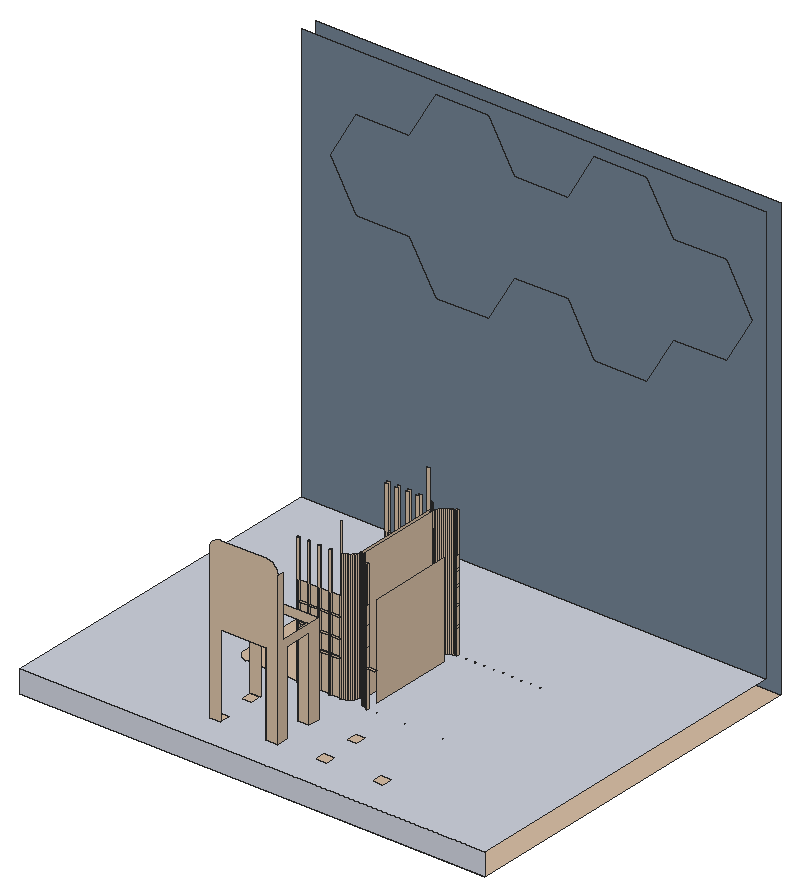
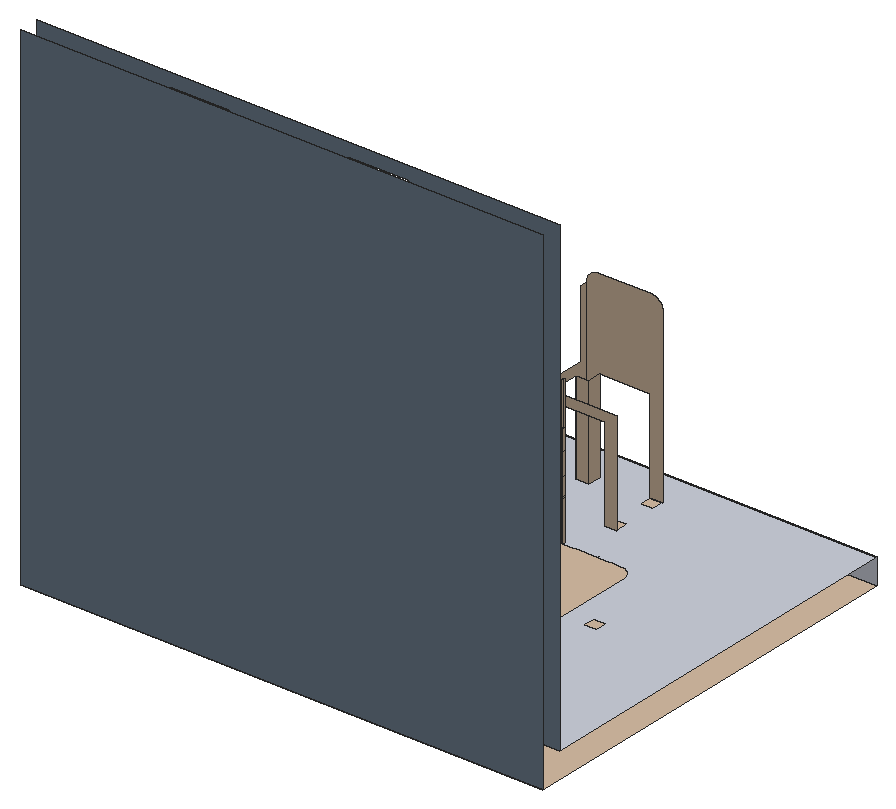
# SketchUp Ruby script. Lengths in inches.
U = 1.inch
M = Sketchup.active_model
def pt(a) = Geom::Point3d.new(a.map { |v| v * U })
def face(e, loops, mat)
  f = e.add_face(loops[0].map { |a| pt(a) })
  loops[1..].each { |l| e.add_face(l.map { |a| pt(a) }).erase! }
  f.material = f.back_material = mat if mat
  f
end
# faces: each face lists its corners as indices into pts; further lists are holes
def faces(e, pts, list, mat = nil) = list.each { |f| face(e, (f[0].is_a?(Array) ? f : [f]).map { |l| l.map { |i| pts[i] } }, mat) }
# xy, xz, yz: faces in a plane at the given z, y or x. An outline is a flat list of corners, or four numbers for a rectangle; further outlines are holes
def ring(l) = l.size == 4 ? [[l[0], l[1]], [l[2], l[1]], [l[2], l[3]], [l[0], l[3]]] : l.each_slice(2).to_a
def flat(e, list, mat, &to3) = list.each { |f| face(e, (f[0].is_a?(Array) ? f : [f]).map { |l| ring(l).map { |u, v| to3.(u, v) } }, mat) }
def xy(e, z, list, mat = nil) = flat(e, list, mat) { |x, y| [x, y, z] }
def xz(e, y, list, mat = nil) = flat(e, list, mat) { |x, z| [x, y, z] }
def yz(e, x, list, mat = nil) = flat(e, list, mat) { |y, z| [x, y, z] }
def lines(e, pts, list) = list.each { |a, b| e.add_line(pt(pts[a]), pt(pts[b])) }
# prism: a flat outline (further loops are holes) pulled along v
def prism(e, loops, v, mat = nil)
  f = face(e, loops, mat); d = Geom::Vector3d.new(v.map { |x| x * U })
  f.pushpull(f.normal.samedirection?(d) ? d.length : -d.length)
end
def box(e, o, s, mat = nil) = prism(e, [[o, [o[0] + s[0], o[1], o[2]], [o[0] + s[0], o[1] + s[1], o[2]], [o[0], o[1] + s[1], o[2]]]], [0, 0, s[2]], mat)
def at(x, y, z, deg = 0) = Geom::Transformation.translation(pt([x, y, z])) * Geom::Transformation.rotation(ORIGIN, Z_AXIS, deg.degrees)
def axes(o, x, y, z) = Geom::Transformation.new([*x, 0, *y, 0, *z, 0, *pt(o).to_a, 1])
def part(name) = M.definitions.add(name)
# library, detail: a bought-in or finely detailed component or shape, given as its bounding box
def library(name, o, s) = part(name).tap { |d| box(d.entities, o, s) }
def detail(e, o, s) = box(e.add_group.entities, o, s)
def put(e, d, t, mat = nil) = e.add_instance(d, t).tap { |i| i.material = mat if mat }
def group(e, t, mat = nil) = e.add_group.tap { |g| g.transformation = t; g.material = mat if mat }.entities
root = M.entities
M.materials.add("[0111_SlateGray]").color = [112, 128, 144]
M.materials.add("[Formica Laminate Light]").color = [213, 189, 164]
M.materials.add("[Marble Carrara Floor Tile]").color = [204, 208, 219]
xy(root,-6.9375,[[214.53,88,358.53,202.625]],"[Formica Laminate Light]")
xy(root,0,[[292.27,124.79,292.63,125.33],[270.89,124.84,271.32,125.33],[274.19,124.84,274.625,125.33],[277.49,124.84,277.93,125.33],[280.8,124.84,281.23,125.33],
  [284.1,124.84,284.53,125.33],[270.69,159.08,271.5,160.01],[273.95,159.08,274.76,160.01],[277.21,159.08,278.02,160.01],[280.47,159.08,281.29,160.01],
  [283.74,159.08,284.55,160.01],[292.34,159.08,293.16,159.77]],"[Formica Laminate Light]")
xy(root,0,[[[214.53,88,358.53,197],[254.37,124.84,254.37,125.33,254.38,125.33,253.95,125.44,253.54,125.6,253.14,125.79,252.77,126.03,252.42,126.3,252.09,126.61,251.81,126.95,251.55,127.3125,251.34,127.7,251.16,128.11,251.03,128.53,250.94,128.96,250.94,156.11,251.04,156.5625,251.21,157.03,251.45,157.47,251.74,157.87,252.09,158.22,252.49,158.52,252.93,158.76,253.4,158.94,253.88,159.05,254.38,159.08,254.38,160.01,255.19,160.01,255.19,159.08,257.64,159.08,257.64,160.01,258.46,160.01,258.46,159.08,260.91,159.08,260.91,160.01,261.72,160.01,261.72,159.08,264.17,159.08,264.17,160.01,264.98,160.01,264.98,159.08,267.43,159.08,267.43,160.01,268.24,160.01,268.24,159.08,270.69,159.08,270.69,160.01,271.5,160.01,271.5,159.08,273.95,159.08,273.95,160.01,274.76,160.01,274.76,159.08,277.21,159.08,277.21,160.01,278.02,160.01,278.02,159.08,280.47,159.08,280.47,160.01,281.29,160.01,281.29,159.08,283.74,159.08,283.74,160.01,284.55,160.01,284.55,159.08,284.99,158.95,285.41,158.77,285.8125,158.55,286.1875,158.28,286.53,157.98,286.83,157.63,287.1,157.26,287.32,156.86,287.49,156.43,287.62,155.99,287.7,155.54,287.72,155.08,287.72,128.96,287.69,128.53,287.62,128.09,287.49,127.67,287.31,127.27,287.08,126.89,286.8125,126.55,286.5,126.23,286.16,125.96,285.78,125.73,285.38,125.55,284.96,125.41,284.53,125.33,284.53,124.84,284.1,124.84,284.1,125.33,281.23,125.33,281.23,124.84,280.8,124.84,280.8,125.33,277.93,125.33,277.93,124.84,277.49,124.84,277.49,125.33,274.625,125.33,274.625,124.84,274.19,124.84,274.19,125.33,271.32,125.33,271.32,124.84,270.89,124.84,270.89,125.33,268.02,125.33,268.02,124.84,267.58,124.84,267.58,125.33,264.71,125.33,264.71,124.84,264.28,124.84,264.28,125.33,261.41,125.33,261.41,124.84,260.98,124.84,260.98,125.33,258.11,125.33,258.11,124.84,257.68,124.84,257.68,125.33,254.81,125.33,254.81,124.84],[297.89,97.95,301.53,101.59],[315.45,97.95,319.1,101.59],[282.83,110.07,286.47,113.72],[282.83,97.95,286.47,101.59],[265.27,97.95,268.91,101.59],[297.89,110.07,301.35,113.72],[265.27,110.07,268.72,113.72],[241.57,147.05,245.21,150.5],[295.2,159.08,296.03,159.77],[318.11,159.08,318.9375,159.77],[292.34,159.08,293.16,159.77],[312.38,159.08,313.21,159.77],[300.93,159.08,301.75,159.77],[309.52,159.08,310.35,159.77],[315.25,159.08,316.07,159.77],[306.66,159.08,307.48,159.77],[298.0625,159.08,298.89,159.77],[303.79,159.08,304.62,159.77],[312.73,124.79,313.09,125.33],[309.81,124.79,310.17,125.33],[315.65,124.79,316.01,125.33],[298.11,124.79,298.47,125.33],[318.58,124.79,318.9375,125.33],[306.88,124.79,307.24,125.33],[295.1875,124.79,295.55,125.33],[301.04,124.79,301.4,125.33],[292.27,124.79,292.63,125.33],[303.96,124.79,304.32,125.33]]],"[Marble Carrara Floor Tile]")
xy(root,7.64,[[271.5,159.08,273.95,160.01],[274.76,159.08,277.21,160.01],[278.02,159.08,280.47,160.01],[281.29,159.08,283.74,160.01]],"[Formica Laminate Light]")
xy(root,8.44,[[271.5,159.08,273.95,160.01],[274.76,159.08,277.21,160.01],[278.02,159.08,280.47,160.01],[281.29,159.08,283.74,160.01]],"[Formica Laminate Light]")
xy(root,11.02,[[271.32,124.84,274.19,125.33],[274.625,124.84,277.49,125.33],[277.93,124.84,280.8,125.33],[281.23,124.84,284.1,125.33]],"[Formica Laminate Light]")
xy(root,11.55,[[292.63,124.79,295.1875,125.33],[271.32,124.84,274.19,125.33],[274.625,124.84,277.49,125.33],[277.93,124.84,280.8,125.33],[281.23,124.84,284.1,125.33]],"[Formica Laminate Light]")
xy(root,15.1,[[271.5,159.08,273.95,160.01],[274.76,159.08,277.21,160.01],[278.02,159.08,280.47,160.01],[281.29,159.08,283.74,160.01]],"[Formica Laminate Light]")
xy(root,15.9,[[271.5,159.08,273.95,160.01],[274.76,159.08,277.21,160.01],[278.02,159.08,280.47,160.01],[281.29,159.08,283.74,160.01]],"[Formica Laminate Light]")
xy(root,16.52,[[271.32,124.84,274.19,125.33],[274.625,124.84,277.49,125.33],[277.93,124.84,280.8,125.33],[281.23,124.84,284.1,125.33]],"[Formica Laminate Light]")
xy(root,20.88,[[271.5,159.08,273.95,160.01],[274.76,159.08,277.21,160.01],[278.02,159.08,280.47,160.01],[281.29,159.08,283.74,160.01]],"[Formica Laminate Light]")
xy(root,21.68,[[271.5,159.08,273.95,160.01],[274.76,159.08,277.21,160.01],[278.02,159.08,280.47,160.01],[281.29,159.08,283.74,160.01]],"[Formica Laminate Light]")
xy(root,22.54,[[271.32,124.84,274.19,125.33],[274.625,124.84,277.49,125.33],[277.93,124.84,280.8,125.33],[281.23,124.84,284.1,125.33]],"[Formica Laminate Light]")
xz(root,88,[[214.53,-6.9375,358.53,0]],"[Marble Carrara Floor Tile]")
xz(root,97.95,[[265.27,0,268.91,0,268.91,25.5625,282.83,25.5625,282.83,0,286.47,0,286.47,46.86,286.41,47.34,286.29,47.8,286.11,48.25,285.88,48.67,285.6,49.05,285.27,49.4,284.9,49.71,284.5,49.97,284.0625,50.17,283.61,50.32,283.14,50.41,282.66,50.4375,268.95,50.4375,268.47,50.41,268,50.3125,267.54,50.16,267.11,49.94,266.71,49.68,266.35,49.36,266.03,48.99,265.76,48.59,265.55,48.16,265.39,47.7,265.3,47.23,265.27,46.75]],"[Formica Laminate Light]")
xz(root,101.59,[[282.83,0,286.47,25.5625]],"[Formica Laminate Light]")
xz(root,110.07,[[282.83,0,286.47,25.5625]],"[Formica Laminate Light]")
xz(root,113.72,[[265.27,0,265.27,28.25,286.47,28.25,286.47,0,282.83,0,282.83,25.5625,268.72,25.5625,268.72,0]],"[Formica Laminate Light]")
xz(root,124.79,[[292.27,0,292.63,40.33]],"[Formica Laminate Light]")
xz(root,124.84,[[270.89,0,271.32,40.33],[274.19,0,274.625,40.33],[277.49,0,277.93,40.33],[280.8,0,281.23,40.33],[271.32,11.02,274.19,11.55],
  [274.625,11.02,277.49,11.55],[277.93,11.02,280.8,11.55],[281.23,11.02,284.1,11.55],[271.32,16.52,274.19,17.06],[274.625,16.52,277.49,17.06],
  [277.93,16.52,280.8,17.06],[281.23,16.52,284.1,17.06],[271.32,22.54,274.19,23.07],[274.625,22.54,277.49,23.07],[277.93,22.54,280.8,23.07],
  [281.23,22.54,284.1,23.07]],"[Formica Laminate Light]")
xz(root,125.33,[[270.89,0,271.32,11.02],[271.32,0,274.19,11.02],[274.19,0,274.625,11.02],[274.625,0,277.49,11.02],[277.49,0,277.93,11.02],
  [277.93,0,280.8,11.02],[280.8,0,281.23,11.02],[281.23,0,284.1,11.02],[284.1,0,284.1,11.02,281.23,11.02,281.23,11.55,284.1,11.55,284.1,49.31,284.53,49.31,284.53,0],[292.27,0,292.32,11.02],
  [292.32,0,292.63,11.02],[270.89,11.02,271.32,40.33],[274.19,11.02,274.625,40.33],[277.49,11.02,277.93,40.33],[280.8,11.02,281.23,40.33],
  [292.27,11.02,292.32,11.55],[292.32,11.02,292.63,11.55],[271.32,11.55,274.19,16.52],[274.625,11.55,277.49,16.52],[277.93,11.55,280.8,16.52],
  [281.23,11.55,284.1,16.52],[292.27,11.55,292.32,40.33],[292.32,11.55,292.63,40.33],[271.32,16.52,274.19,22.54],[274.625,16.52,277.49,22.54],
  [277.93,16.52,280.8,22.54],[281.23,16.52,284.1,22.54],[271.32,22.54,274.19,28.4],[274.625,22.54,277.49,28.4],[277.93,22.54,280.8,28.4],
  [281.23,22.54,284.1,28.4]],"[Formica Laminate Light]")
xz(root,159.08,[[270.69,0,271.5,40.33],[271.5,0,273.95,7.64],[273.95,0,274.76,40.33],[274.76,0,277.21,7.64],[277.21,0,278.02,40.33],
  [278.02,0,280.47,7.64],[280.47,0,281.29,40.33],[281.29,0,283.74,7.64],[283.74,0,284.55,0,284.55,49.31,283.74,49.31,283.74,8.44,281.29,8.44,281.29,7.64,283.74,7.64],[292.34,0,292.97,40.33],
  [292.97,0,293.16,40.33],[271.5,8.44,273.95,15.1],[274.76,8.44,277.21,15.1],[278.02,8.44,280.47,15.1],[281.29,8.44,283.74,15.1],
  [271.5,15.1,273.95,15.9],[274.76,15.1,277.21,15.9],[278.02,15.1,280.47,15.9],[281.29,15.1,283.74,15.9],[271.5,15.9,273.95,20.88],
  [274.76,15.9,277.21,20.88],[278.02,15.9,280.47,20.88],[281.29,15.9,283.74,20.88],[271.5,20.88,273.95,21.68],[274.76,20.88,277.21,21.68],
  [278.02,20.88,280.47,21.68],[281.29,20.88,283.74,21.68],[271.5,21.68,273.95,26.83],[274.76,21.68,277.21,26.83],[278.02,21.68,280.47,26.83],
  [281.29,21.68,283.74,26.83]],"[Formica Laminate Light]")
xz(root,159.77,[[292.34,0,293.16,40.33]],"[Formica Laminate Light]")
xz(root,160.01,[[270.69,0,271.5,40.33],[273.95,0,274.76,40.33],[277.21,0,278.02,40.33],[280.47,0,281.29,40.33],[271.5,7.64,273.95,8.44],
  [274.76,7.64,277.21,8.44],[278.02,7.64,280.47,8.44],[281.29,7.64,283.74,8.44],[271.5,15.1,273.95,15.9],[274.76,15.1,277.21,15.9],
  [278.02,15.1,280.47,15.9],[281.29,15.1,283.74,15.9],[271.5,20.88,273.95,21.68],[274.76,20.88,277.21,21.68],[278.02,20.88,280.47,21.68],
  [281.29,20.88,283.74,21.68]],"[Formica Laminate Light]")
xz(root,197,[[[214.53,0,358.53,129.75],[256.11,69.64,247.92,83.83,231.54,83.83,223.35,98.02,231.54,112.21,247.92,112.21,256.11,126.39,272.5,126.39,280.6875,112.21,297.07,112.21,305.26,126.39,321.64,126.39,329.84,112.21,346.22,112.21,354.41,98.02,346.22,83.83,329.84,83.83,321.64,69.64,305.26,69.64,297.07,83.83,280.6875,83.83,272.5,69.64]]],"[0111_SlateGray]")
xz(root,202.625,[[214.53,-6.9375,358.53,129.75]],"[0111_SlateGray]")
yz(root,270.69,[[159.08,0,160.01,7.64],[159.08,20.88,160.01,21.68],[159.08,21.68,160.01,26.83]],"[Formica Laminate Light]")
yz(root,270.89,[[124.84,0,125.33,11.02],[124.84,11.02,125.33,11.55],[124.84,11.55,125.33,16.52],[124.84,16.52,125.33,22.54],[124.84,22.54,125.33,28.4]],"[Formica Laminate Light]")
yz(root,271.32,[[124.84,0,125.33,11.02],[124.84,11.02,125.33,11.55],[124.84,11.55,125.33,16.52],[124.84,16.52,125.33,22.54],[124.84,22.54,125.33,28.4]],"[Formica Laminate Light]")
yz(root,271.5,[[159.08,0,160.01,7.64],[159.08,7.64,160.01,8.44],[159.08,8.44,160.01,15.1],[159.08,15.1,160.01,15.9],[159.08,15.9,160.01,20.88],
  [159.08,20.88,160.01,21.68],[159.08,21.68,160.01,26.83]],"[Formica Laminate Light]")
yz(root,273.95,[[159.08,0,160.01,7.64],[159.08,7.64,160.01,8.44],[159.08,8.44,160.01,15.1],[159.08,15.1,160.01,15.9],[159.08,15.9,160.01,20.88],
  [159.08,20.88,160.01,21.68],[159.08,21.68,160.01,26.83]],"[Formica Laminate Light]")
yz(root,274.19,[[124.84,0,125.33,11.02],[124.84,11.02,125.33,11.55],[124.84,11.55,125.33,16.52],[124.84,16.52,125.33,22.54],[124.84,22.54,125.33,28.4]],"[Formica Laminate Light]")
yz(root,274.625,[[124.84,0,125.33,11.02],[124.84,11.02,125.33,11.55],[124.84,11.55,125.33,16.52],[124.84,16.52,125.33,22.54],[124.84,22.54,125.33,28.4]],"[Formica Laminate Light]")
yz(root,274.76,[[159.08,0,160.01,7.64],[159.08,7.64,160.01,8.44],[159.08,8.44,160.01,15.1],[159.08,15.1,160.01,15.9],[159.08,15.9,160.01,20.88],
  [159.08,20.88,160.01,21.68],[159.08,21.68,160.01,26.83]],"[Formica Laminate Light]")
yz(root,277.21,[[159.08,0,160.01,7.64],[159.08,7.64,160.01,8.44],[159.08,8.44,160.01,15.1],[159.08,15.1,160.01,15.9],[159.08,15.9,160.01,20.88],
  [159.08,20.88,160.01,21.68],[159.08,21.68,160.01,26.83]],"[Formica Laminate Light]")
yz(root,277.49,[[124.84,0,125.33,11.02],[124.84,11.02,125.33,11.55],[124.84,11.55,125.33,16.52],[124.84,16.52,125.33,22.54],[124.84,22.54,125.33,28.4]],"[Formica Laminate Light]")
yz(root,277.93,[[124.84,0,125.33,11.02],[124.84,11.02,125.33,11.55],[124.84,11.55,125.33,16.52],[124.84,16.52,125.33,22.54],[124.84,22.54,125.33,28.4]],"[Formica Laminate Light]")
yz(root,278.02,[[159.08,0,160.01,7.64],[159.08,7.64,160.01,8.44],[159.08,8.44,160.01,15.1],[159.08,15.1,160.01,15.9],[159.08,15.9,160.01,20.88],
  [159.08,20.88,160.01,21.68],[159.08,21.68,160.01,26.83]],"[Formica Laminate Light]")
yz(root,280.47,[[159.08,0,160.01,7.64],[159.08,7.64,160.01,8.44],[159.08,8.44,160.01,15.1],[159.08,15.1,160.01,15.9],[159.08,15.9,160.01,20.88],
  [159.08,20.88,160.01,21.68],[159.08,21.68,160.01,26.83]],"[Formica Laminate Light]")
yz(root,280.8,[[124.84,0,125.33,11.02],[124.84,11.02,125.33,11.55],[124.84,11.55,125.33,16.52],[124.84,16.52,125.33,22.54],[124.84,22.54,125.33,28.4]],"[Formica Laminate Light]")
yz(root,281.23,[[124.84,0,125.33,11.02],[124.84,11.02,125.33,11.55],[124.84,11.55,125.33,16.52],[124.84,16.52,125.33,22.54],[124.84,22.54,125.33,28.4]],"[Formica Laminate Light]")
yz(root,281.29,[[159.08,0,160.01,7.64],[159.08,7.64,160.01,8.44],[159.08,8.44,160.01,15.1],[159.08,15.1,160.01,15.9],[159.08,15.9,160.01,20.88],
  [159.08,20.88,160.01,21.68],[159.08,21.68,160.01,26.83]],"[Formica Laminate Light]")
yz(root,282.83,[[97.95,0,101.59,25.5625],[110.07,0,113.72,25.5625]],"[Formica Laminate Light]")
yz(root,283.74,[[159.08,0,160.01,7.64],[159.08,8.44,160.01,15.1],[159.08,15.1,160.01,15.9],[159.08,15.9,160.01,20.88],[159.08,20.88,160.01,21.68],
  [159.08,21.68,160.01,26.83]],"[Formica Laminate Light]")
yz(root,284.1,[[124.84,0,125.33,11.02],[124.84,11.55,125.33,16.52],[124.84,16.52,125.33,22.54],[124.84,22.54,125.33,28.4]],"[Formica Laminate Light]")
yz(root,284.55,[[128.96,0,155.08,28.69]],"[Formica Laminate Light]")
yz(root,286.47,[[97.95,0,101.59,0,101.59,25.5625,110.07,25.5625,110.07,0,113.72,0,113.72,28.25,99.82,28.25,99.82,46.86,97.95,46.86]],"[Formica Laminate Light]")
yz(root,287.72,[[128.96,0,155.08,40.33]],"[Formica Laminate Light]")
yz(root,288.6,[[129.05,0,155.08,40.33]],"[Formica Laminate Light]")
yz(root,292.27,[[124.79,0,125.33,40.33]],"[Formica Laminate Light]")
yz(root,292.34,[[128.96,0,155.08,28.69],[159.08,0,159.77,40.33]],"[Formica Laminate Light]")
yz(root,292.63,[[124.79,0,125.33,11.02],[124.79,11.02,125.33,11.55],[124.79,11.55,125.33,17.15],[124.79,17.15,125.33,23.36],[124.79,23.36,125.33,28.96]],"[Formica Laminate Light]")
yz(root,293.16,[[159.08,0,159.77,7.64],[159.08,7.64,159.77,8.44],[159.08,8.44,159.77,13.77],[159.08,13.77,159.77,14.57],[159.08,14.57,159.77,19.01],
  [159.08,19.01,159.77,19.8125],[159.08,19.8125,159.77,23.54],[159.08,23.54,159.77,24.34],[159.08,24.34,159.77,27.9]],"[Formica Laminate Light]")
p = [[284.53,125.33,40.33],[284.53,125.33,0],[284.96,125.41,0],[284.96,125.41,40.33],[291.83,125.36,40.33],[291.83,125.36,0],
  [292.32,125.33,0],[292.32,125.33,11.02],[292.32,125.33,11.55],[292.32,125.33,40.33],[285.38,125.55,0],[285.38,125.55,40.33],
  [291.36,125.45,40.33],[291.36,125.45,0],[285.78,125.73,0],[285.78,125.73,40.33],[290.9,125.61,40.33],[290.9,125.61,0],
  [290.46,125.83,40.33],[290.46,125.83,0],[286.16,125.96,0],[286.16,125.96,40.33],[290.05,126.1,40.33],[290.05,126.1,0],
  [286.5,126.23,0],[286.5,126.23,40.33],[289.6875,126.42,40.33],[289.6875,126.42,0],[286.8125,126.55,0],[286.8125,126.55,40.33],
  [289.37,126.78,40.33],[289.37,126.78,0],[287.08,126.89,0],[287.08,126.89,40.33],[289.1,127.1875,40.33],[289.1,127.1875,0],
  [287.31,127.27,0],[287.31,127.27,40.33],[288.88,127.62,40.33],[288.88,127.62,0],[287.49,127.67,0],[287.49,127.67,40.33],
  [288.73,128.08,40.33],[288.73,128.08,0],[287.62,128.09,0],[287.62,128.09,40.33],[287.69,128.53,0],[287.69,128.53,40.33],
  [288.63,128.5625,40.33],[288.63,128.5625,0],[287.72,128.96,0],[287.72,128.96,40.33],[288.6,129.05,40.33],[288.6,129.05,0],
  [287.72,155.08,40.33],[287.72,155.08,0],[287.7,155.54,0],[287.7,155.54,40.33],[288.63,155.58,40.33],[288.63,155.58,0],
  [288.6,155.08,0],[288.6,155.08,40.33],[287.62,155.99,0],[287.62,155.99,40.33],[288.72,156.07,40.33],[288.72,156.07,0],
  [287.49,156.43,0],[287.49,156.43,40.33],[288.88,156.55,40.33],[288.88,156.55,0],[287.32,156.86,0],[287.32,156.86,40.33],
  [289.09,157.01,40.33],[289.09,157.01,0],[287.1,157.26,0],[287.1,157.26,40.33],[289.36,157.43,40.33],[289.36,157.43,0],
  [286.83,157.63,0],[286.83,157.63,40.33],[289.68,157.82,40.33],[289.68,157.82,0],[286.53,157.98,0],[286.53,157.98,40.33],
  [290.04,158.16,40.33],[290.04,158.16,0],[286.1875,158.28,0],[286.1875,158.28,40.33],[290.45,158.46,40.33],[290.45,158.46,0],
  [285.8125,158.55,0],[285.8125,158.55,40.33],[290.89,158.7,40.33],[290.89,158.7,0],[285.41,158.77,0],[285.41,158.77,40.33],
  [291.35,158.89,40.33],[291.35,158.89,0],[284.99,158.95,0],[284.99,158.95,40.33],[291.84,159.02,40.33],[291.84,159.02,0],
  [284.55,159.08,0],[284.55,159.08,40.33],[292.34,159.08,40.33],[292.34,159.08,0],[284.53,124.84,0],[284.53,124.84,40.33],
  [284.55,160.01,0],[284.55,160.01,40.33]]
faces(root,p,[[0,1,2,3],[4,5,6,7,8,9],[3,2,10,11],[12,13,5,4],[11,10,14,15],[16,17,13,12],[18,19,17,16],[15,14,20,21],
  [22,23,19,18],[21,20,24,25],[26,27,23,22],[25,24,28,29],[30,31,27,26],[29,28,32,33],[34,35,31,30],[33,32,36,37],
  [38,39,35,34],[37,36,40,41],[42,43,39,38],[41,40,44,45],[45,44,46,47],[48,49,43,42],[47,46,50,51],[52,53,49,48],
  [54,55,56,57],[58,59,60,61],[57,56,62,63],[64,65,59,58],[63,62,66,67],[68,69,65,64],[67,66,70,71],[72,73,69,68],
  [71,70,74,75],[76,77,73,72],[75,74,78,79],[80,81,77,76],[79,78,82,83],[84,85,81,80],[83,82,86,87],[88,89,85,84],
  [87,86,90,91],[92,93,89,88],[91,90,94,95],[96,97,93,92],[95,94,98,99],[100,101,97,96],[99,98,102,103],[104,105,101,100]],"[Formica Laminate Light]")
lines(root,p,[[106,107],[108,109]])
